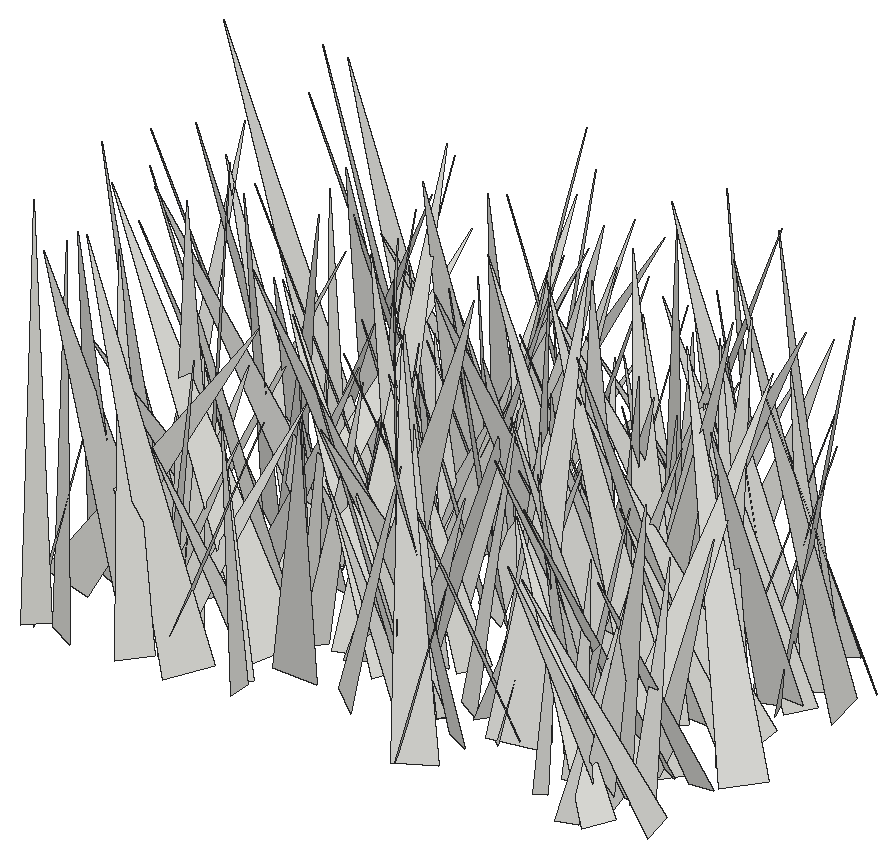
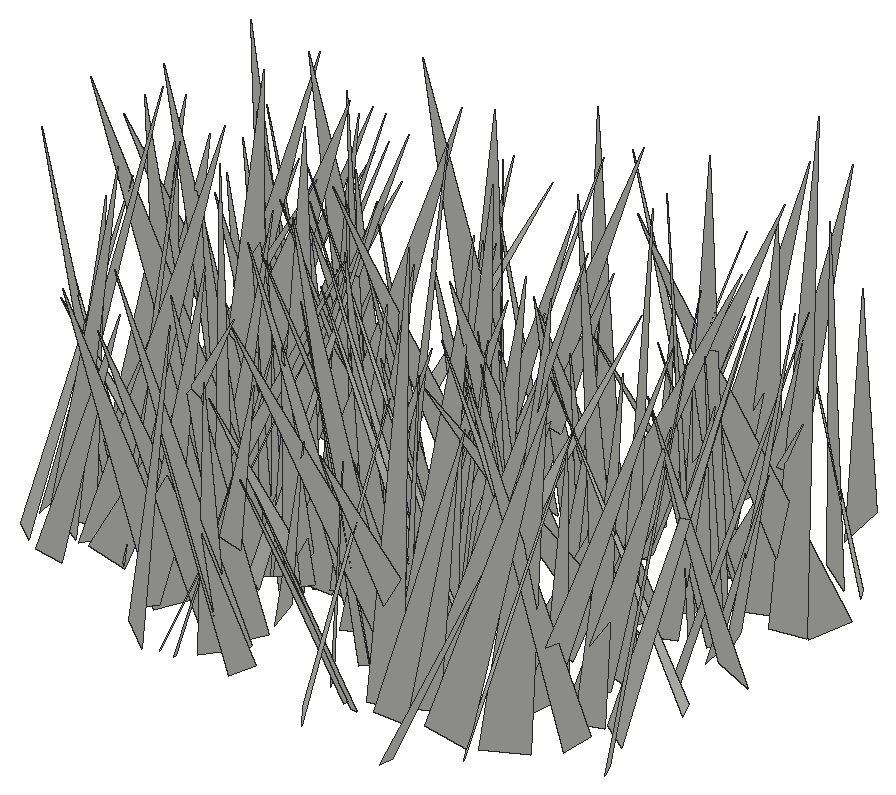
# SketchUp Ruby script. Lengths in inches.
U = 1.inch
M = Sketchup.active_model
def pt(a) = Geom::Point3d.new(a.map { |v| v * U })
def face(e, loops, mat)
  f = e.add_face(loops[0].map { |a| pt(a) })
  loops[1..].each { |l| e.add_face(l.map { |a| pt(a) }).erase! }
  f.material = f.back_material = mat if mat
  f
end
# faces: each face lists its corners as indices into pts; further lists are holes
def faces(e, pts, list, mat = nil) = list.each { |f| face(e, (f[0].is_a?(Array) ? f : [f]).map { |l| l.map { |i| pts[i] } }, mat) }
# xy, xz, yz: faces in a plane at the given z, y or x. An outline is a flat list of corners, or four numbers for a rectangle; further outlines are holes
def ring(l) = l.size == 4 ? [[l[0], l[1]], [l[2], l[1]], [l[2], l[3]], [l[0], l[3]]] : l.each_slice(2).to_a
def flat(e, list, mat, &to3) = list.each { |f| face(e, (f[0].is_a?(Array) ? f : [f]).map { |l| ring(l).map { |u, v| to3.(u, v) } }, mat) }
def xy(e, z, list, mat = nil) = flat(e, list, mat) { |x, y| [x, y, z] }
def xz(e, y, list, mat = nil) = flat(e, list, mat) { |x, z| [x, y, z] }
def yz(e, x, list, mat = nil) = flat(e, list, mat) { |y, z| [x, y, z] }
def lines(e, pts, list) = list.each { |a, b| e.add_line(pt(pts[a]), pt(pts[b])) }
# prism: a flat outline (further loops are holes) pulled along v
def prism(e, loops, v, mat = nil)
  f = face(e, loops, mat); d = Geom::Vector3d.new(v.map { |x| x * U })
  f.pushpull(f.normal.samedirection?(d) ? d.length : -d.length)
end
def box(e, o, s, mat = nil) = prism(e, [[o, [o[0] + s[0], o[1], o[2]], [o[0] + s[0], o[1] + s[1], o[2]], [o[0], o[1] + s[1], o[2]]]], [0, 0, s[2]], mat)
def at(x, y, z, deg = 0) = Geom::Transformation.translation(pt([x, y, z])) * Geom::Transformation.rotation(ORIGIN, Z_AXIS, deg.degrees)
def axes(o, x, y, z) = Geom::Transformation.new([*x, 0, *y, 0, *z, 0, *pt(o).to_a, 1])
def part(name) = M.definitions.add(name)
# library, detail: a bought-in or finely detailed component or shape, given as its bounding box
def library(name, o, s) = part(name).tap { |d| box(d.entities, o, s) }
def detail(e, o, s) = box(e.add_group.entities, o, s)
def put(e, d, t, mat = nil) = e.add_instance(d, t).tap { |i| i.material = mat if mat }
def group(e, t, mat = nil) = e.add_group.tap { |g| g.transformation = t; g.material = mat if mat }.entities
root = M.entities
c1 = part("fur_instance\#9")
p = [[0.8125,0,1.79],[0.67,-0.02,1.48],[0,-0.11,0],[0,0.11,0]]
faces(c1.entities,p,[[0,1,2,3]])
put(root,c1,axes([89.75,154.68,-28.22],[3.15545,2.01724,0.79775],[2.15051,-3.09372,-0.68323],[-0.2846,-1.01105,3.6823]))
put(root,c1,axes([95.03,153.1,-27.1],[-6.05277,2.56522,0.71834],[2.46544,6.06973,-0.90131],[1.00895,0.55714,6.51184]))
put(root,c1,axes([95.66,155,-28.22],[-6.02527,4.37662,1.94606],[4.73834,5.90349,1.39383],[0.70004,-2.28907,7.31546]))
put(root,c1,axes([98.42,156.88,-28.22],[1.84605,-6.6162,0.27609],[-6.51912,-1.76548,1.28157],[1.16252,0.60597,6.74831]))
put(root,c1,axes([93.76,156.59,-28.22],[6.81977,1.54998,0.06465],[1.44583,-6.24479,-2.79788],[0.56233,-2.74155,6.40965]))
put(root,c1,axes([104.08,154.99,-28.22],[3.27913,1.40298,0.59687],[1.4938,-3.23974,-0.59158],[-0.30522,-0.78299,3.51725]))
put(root,c1,axes([91.07,154.34,-28.22],[3.04497,5.63186,2.55497],[5.93211,-3.46487,0.56775],[-1.7481,-1.94792,6.3771]))
put(root,c1,axes([91.22,152.89,-27.1],[-6.67208,0.88571,0.68005],[0.61302,6.34873,-2.25421],[0.93335,2.16166,6.3419]))
put(root,c1,axes([113.36,156.39,-28.22],[-4.90231,-0.23018,0.15933],[-0.18525,4.76264,1.18065],[0.20988,-1.17272,4.76358]))
put(root,c1,axes([111.52,156.59,-28.22],[-4.7933,-0.97536,0.74224],[-0.77682,4.73507,1.20565],[0.94805,-1.05153,4.74061]))
put(root,c1,axes([97.63,155.1,-28.22],[-4.49863,-0.46507,1.40367],[-0.60193,4.68178,-0.37796],[1.35065,0.53749,4.50678]))
put(root,c1,axes([91.66,157.73,-28.22],[5.20163,-5.29224,1.8402],[-4.95757,-5.51713,-1.85336],[-2.61089,-0.0677,7.18539]))
put(root,c1,axes([96.51,157.05,-28.22],[-4.25051,-1.02119,0.70994],[-0.79222,4.17184,1.25768],[0.95876,-1.08007,4.18663]))
put(root,c1,axes([89.99,158.09,-28.22],[-1.25565,-8.18969,1.33935],[-8.04493,1.53362,1.83538],[2.03567,1.00923,8.07955]))
put(root,c1,axes([104.86,154.85,-28.22],[-2.95923,6.17255,1.7602],[6.41346,2.92118,0.53848],[0.25723,-1.82266,6.82403]))
put(root,c1,axes([104.99,156.82,-28.22],[-2.87551,-4.98025,1.4124],[-5.17006,2.84441,-0.49611],[0.26119,1.47404,5.72934]))
put(root,c1,axes([100.61,156.65,-28.22],[3.06956,3.90435,1.71137],[4.25532,-2.68017,-1.51785],[0.25498,-2.27325,4.72887]))
put(root,c1,axes([111.77,155.4375,-28.22],[-3.00277,4.1066,0.06153],[3.92812,2.84936,1.52829],[-1.19912,-0.94951,4.85234]))
put(root,c1,axes([110.73,157.375,-28.22],[1.26894,-6.32164,1.3833],[-6.3592,-0.957,1.46001],[1.19887,1.6149,6.28026]))
put(root,c1,axes([111.05,156.16,-28.22],[4.20018,-2.603,1.54886],[-2.85846,-4.28223,0.55487],[-1.0019,1.30501,4.91012]))
put(root,c1,axes([94.16,155.69,-28.22],[4.52412,1.43506,1.852],[1.32361,-4.8885,0.5546],[-1.93323,0.01133,4.71375]))
put(root,c1,axes([93.89,156.42,-28.22],[-2.52559,2.65872,0.46687],[2.62617,2.27215,1.26725],[-0.62447,-1.19747,3.44114]))
put(root,c1,axes([97.36,155.55,-28.22],[-3.44021,1.49763,0.22694],[1.46636,3.43395,-0.43273],[0.37973,0.30751,3.72702]))
put(root,c1,axes([109.33,157.41,-28.22],[-1.75963,-5.21212,1.71135],[-5.46295,1.82898,-0.04671],[0.50104,1.63703,5.50093]))
put(root,c1,axes([103.04,157.14,-28.22],[-5.74367,-4.09689,1.01684],[-4.21686,5.6466,-1.0688],[0.19121,1.46278,6.97366]))
put(root,c1,axes([110.91,154.9,-28.22],[-3.77654,1.99621,0.89861],[1.50689,3.67022,-1.82025],[1.58796,1.26459,3.86442]))
put(root,c1,axes([89.07,157.1,-28.22],[3.63581,-6.29578,1.08718],[-5.74464,-2.67402,3.72648],[2.79605,2.69271,6.24254]))
put(root,c1,axes([92.64,157.16,-28.22],[2.90459,3.11145,0.76807],[3.13189,-2.53582,-1.57117],[0.67994,-1.61126,3.9559]))
put(root,c1,axes([109.1,157.25,-28.22],[4.01593,3.70117,1.52807],[3.99587,-3.8439,-1.19115],[-0.25835,-1.92018,5.32987]))
put(root,c1,axes([111.21,159.3,-28.22],[-1.38983,-5.84462,0.0201],[-5.82782,1.38425,-0.46046],[-0.44334,0.12603,5.98992]))
put(root,c1,axes([109.51,157.06,-28.22],[0.95056,-3.70171,1.6828],[-4.06505,-0.90725,0.30052],[-0.09921,1.70654,3.80998]))
put(root,c1,axes([94.23,155.71,-28.22],[1.65691,4.63189,0.02775],[4.518,-1.60961,-1.09423],[1.0212,-0.39403,4.79608]))
put(root,c1,axes([102.22,157.55,-28.22],[-3.97846,-0.22397,0.26493],[-0.21326,3.98441,0.16592],[0.27363,-0.15114,3.9813]))
put(root,c1,axes([103.54,157.51,-28.22],[-1.39517,3.65073,1.37856],[3.73252,0.82124,1.60268],[-1.13865,-1.78115,3.56451]))
put(root,c1,axes([97.07,157.6,-28.22],[-7.15301,3.97515,0.71331],[4.02795,6.91641,1.848],[-0.2937,-1.95899,7.97197]))
put(root,c1,axes([112.79,159.31,-28.22],[-0.25255,-4.7231,0.0991],[-4.68784,0.23828,-0.59045],[-0.58449,0.12972,4.69284]))
put(root,c1,axes([112.24,157.03,-28.22],[0.04059,4.23783,1.33242],[4.44047,0.00019,-0.13586],[0.12965,-1.33303,4.23585]))
put(root,c1,axes([109.14,155.79,-28.22],[1.37607,4.21587,0.41156],[3.82506,-1.42264,1.78368],[-1.81985,0.19763,4.06025]))
put(root,c1,axes([106.23,158.34,-28.22],[-5.23491,-4.53939,0.15815],[-4.43832,5.06084,-1.65066],[-0.96564,1.34804,6.72946]))
put(root,c1,axes([103.45,157.3125,-28.22],[-4.02288,2.74208,1.38872],[2.85785,4.17888,0.02734],[1.13147,-0.80565,4.86845]))
put(root,c1,axes([108.68,159.2,-28.22],[3.89618,-1.88557,1.1779],[-1.51971,-3.99347,-1.36592],[-1.62275,-0.78732,4.1073]))
put(root,c1,axes([93,158.62,-28.22],[6.49174,-3.69034,2.54193],[-3.75607,-6.92147,-0.45599],[-2.44375,0.83512,7.45341]))
put(root,c1,axes([110.06,158.83,-28.22],[-6.30832,-1.1114,1.05664],[-1.00602,6.37534,0.69964],[1.15742,-0.51611,6.36715]))
put(root,c1,axes([94.56,156.49,-28.22],[-4.63028,1.37895,0.71291],[1.15549,4.55932,-1.31404],[1.03661,1.07721,4.64912]))
put(root,c1,axes([110.44,159.28,-28.22],[-1.67937,-5.43767,0.87836],[-5.25266,1.30456,-1.96667],[-1.65811,1.37475,5.34049]))
put(root,c1,axes([101.4,158.98,-28.22],[3.13596,-3.23192,0.2957],[-3.22644,-3.06024,0.76944],[0.35051,0.74607,4.43707]))
put(root,c1,axes([99.68,159.16,-28.22],[6.25642,-5.32962,1.03257],[-5.42827,-6.12142,1.29455],[0.06986,1.65444,8.11614]))
put(root,c1,axes([100.4,161.69,-28.22],[5.3138,-2.81187,1.14067],[-1.98861,-4.96443,-2.9739],[-2.29198,-2.2118,5.22484]))
put(root,c1,axes([105.83,157.65,-28.22],[2.60004,3.22909,0.64132],[3.22546,-2.66223,0.32783],[-0.65933,-0.2899,4.13277]))
put(root,c1,axes([100.03,161.35,-28.22],[-0.28332,-7.79704,0.77926],[-7.68212,0.12267,-1.56569],[-1.54472,0.82004,7.64347]))
put(root,c1,axes([111.26,158.86,-28.22],[4.23339,-1.74729,1.15695],[-1.93705,-4.25778,0.65751],[-0.79963,1.0637,4.53236]))
put(root,c1,axes([100.9,158.96,-28.22],[4.97701,4.02381,2.97396],[4.34378,-5.5566,0.24873],[-2.48337,-1.65505,6.3953]))
put(root,c1,axes([96.49,159.06,-28.22],[-7.32124,-3.15954,0.71739],[-3.23761,7.2018,-1.32279],[0.12329,1.49974,7.86343]))
put(root,c1,axes([97.66,158.77,-28.22],[4.38322,-1.64948,1.59394],[-1.93146,-4.50849,0.64578],[-1.2373,1.19448,4.63858]))
put(root,c1,axes([106.49,157.76,-28.22],[-2.78975,7.45432,2.27613],[7.61508,3.12201,-0.8911],[1.66081,-1.79348,7.90921]))
put(root,c1,axes([107,158.4,-28.22],[-1.61358,3.38665,0.61033],[3.4322,1.63258,0.01498],[0.24881,-0.55751,3.75138]))
put(root,c1,axes([90.68,162.89,-28.22],[-5.2943,-3.28141,1.0592],[-2.29433,4.80125,3.40634],[2.57403,-2.46971,5.21479]))
put(root,c1,axes([104,158.61,-28.22],[2.52877,4.50107,1.40807],[4.66336,-2.62485,0.01569],[-0.70386,-1.21962,5.16276]))
put(root,c1,axes([104.61,160.28,-28.22],[3.51068,-4.45404,1.06123],[-4.56743,-3.50052,0.41776],[-0.32136,1.09429,5.65587]))
put(root,c1,axes([101.22,160.06,-28.22],[1.40139,-5.88916,2.09043],[-6.21682,-1.53152,-0.14692],[-0.635,1.99706,6.05182]))
put(root,c1,axes([104.79,158.55,-28.22],[5.00649,-0.69371,1.01239],[-0.92226,-4.93206,1.18126],[-0.80969,1.32843,4.91435]))
put(root,c1,axes([100.7,159.03,-28.22],[-4.99082,4.3261,0.4502],[4.29852,4.80129,1.51542],[-0.66378,-1.43477,6.4286]))
put(root,c1,axes([96.7,159.86,-28.22],[-3.86454,-2.68359,1.87384],[-2.96857,4.09497,-0.25773],[1.3786,1.29506,4.69786]))
put(root,c1,axes([111.6,159.08,-28.22],[-2.9065,7.574,1.65107],[7.44857,2.24028,2.83534],[-2.14716,-2.4809,7.60092]))
put(root,c1,axes([92.16,160.19,-28.22],[6.26613,3.81902,2.82967],[4.24719,-6.60086,-0.4964],[-2.13385,-1.92357,7.3214]))
put(root,c1,axes([91.94,159.12,-28.22],[-4.86729,-1.78674,2.25978],[-2.35287,5.02555,-1.09424],[1.66225,1.88173,5.06809]))
put(root,c1,axes([96.64,159.73,-28.22],[4.11345,0.18865,1.81103],[0.00918,-4.47631,0.44541],[-1.8208,0.4036,4.09361]))
put(root,c1,axes([91.16,160.11,-28.22],[0.33455,3.97904,1.71347],[4.11253,0.24873,-1.38056],[1.36232,-1.72801,3.74683]))
put(root,c1,axes([93.95,160.3,-28.22],[4.93305,-2.19664,0.15391],[-2.18894,-4.85066,0.92924],[0.23965,0.9109,5.31946]))
put(root,c1,axes([90.83,159.85,-28.22],[-6.73527,-1.87686,1.53677],[-2.12146,6.75676,-1.04577],[1.17629,1.43931,6.91323]))
put(root,c1,axes([110.32,162.51,-28.22],[-0.93689,-7.58778,0.99671],[-7.63501,0.85799,-0.64504],[-0.52389,1.06539,7.61814]))
put(root,c1,axes([102.55,160.74,-28.22],[-3.29735,3.76242,1.32483],[3.9802,2.99017,1.41439],[-0.2628,-1.92005,4.79874]))
put(root,c1,axes([112.62,161.26,-28.22],[-4.62797,0.36048,0.06702],[0.36662,4.56134,0.78248],[0.00509,-0.78533,4.57556]))
put(root,c1,axes([110.4375,158.32,-28.22],[-1.75958,6.89289,0.89816],[6.66639,1.93582,-1.79628],[1.96924,-0.39424,6.88342]))
put(root,c1,axes([90.89,160.72,-28.22],[-3.86057,-0.50737,0.50019],[-0.53854,3.88252,-0.21837],[0.46646,0.28336,3.88764]))
put(root,c1,axes([102.22,158.06,-28.22],[7.12647,2.20024,1.82821],[1.44023,-6.99989,2.8102],[-2.47167,2.26505,6.90872]))
put(root,c1,axes([108.63,160.82,-28.22],[-8.06825,0.70999,0.37952],[0.71569,8.07597,0.10667],[0.36866,-0.13964,8.09873]))
put(root,c1,axes([95.95,162.07,-28.22],[-0.05824,-3.81958,0.55077],[-3.85535,0.08183,0.15984],[0.16986,0.54776,3.81668]))
put(root,c1,axes([104.04,161.77,-28.22],[7.07527,1.73735,2.55738],[2.12787,-7.36989,-0.88027],[-2.24293,-1.5114,7.23207]))
put(root,c1,axes([92.92,160.8,-28.22],[-3.33055,3.67395,0.98734],[3.8043,3.21801,0.85849],[0.0046,-1.30837,4.884]))
put(root,c1,axes([104.76,161.06,-28.22],[1.88047,-2.78184,1.95652],[-3.20631,-2.19563,-0.04014],[-1.13412,1.59479,3.35756]))
put(root,c1,axes([113.75,160.25,-28.22],[-4.84886,5.21937,0.60309],[5.25064,4.78392,0.8135],[-0.19034,-0.99462,7.07753]))
put(root,c1,axes([112.51,162.64,-28.22],[-6.49837,1.01991,0.13564],[1.01971,6.26851,1.71854],[-0.13717,-1.71841,6.34946]))
put(root,c1,axes([106.7,161.48,-28.22],[4.67154,-2.82363,0.84685],[-2.94301,-4.55853,1.0353],[-0.16964,1.32674,5.35951]))
put(root,c1,axes([95.23,163.375,-28.22],[0.24896,-7.3468,1.55373],[-6.97419,-0.80255,-2.67734],[-2.78393,1.35351,6.84612]))
put(root,c1,axes([106.46,163.44,-28.22],[-0.95692,-4.60949,0.0097],[-4.59629,0.95343,-0.35816],[-0.34872,0.08227,4.69412]))
put(root,c1,axes([91.27,164.24,-28.22],[-5.06426,-4.56399,0.84014],[-4.29824,5.08189,1.69768],[1.74956,-0.72593,6.60262]))
put(root,c1,axes([103.72,165.08,-28.22],[1.8393,-7.94223,0.20343],[-7.82957,-1.84746,-1.33722],[-1.34842,-0.10629,8.04201]))
put(root,c1,axes([91.95,163.83,-28.22],[-3.33298,-6.74445,1.96036],[-6.484,3.7887,2.01069],[2.69971,0.77298,7.24938]))
put(root,c1,axes([100.91,164.12,-28.22],[-3.9717,-6.10655,1.7462],[-5.81347,4.32471,1.90107],[2.55787,0.34722,7.03209]))
put(root,c1,axes([109.38,161.49,-28.22],[-5.36752,5.77658,2.45123],[6.12108,5.53013,0.37117],[1.38195,-2.05828,7.87664]))
put(root,c1,axes([100.49,161.9375,-28.22],[-0.11529,-4.79427,2.44231],[-5.06003,0.9271,1.58106],[1.8292,2.26244,4.52754]))
put(root,c1,axes([92.68,163.7,-28.22],[7.66875,0.29762,1.40281],[0.64374,-7.5341,-1.92071],[-1.28143,-2.00373,7.43029]))
put(root,c1,axes([104.48,159.58,-28.22],[3.19327,6.60837,0.52108],[6.51338,-3.23542,1.11669],[-1.23207,0.02336,7.254]))
put(root,c1,axes([97.54,162.26,-28.22],[3.79573,2.84609,1.46317],[3.05532,-3.89817,-0.34352],[-0.95191,-1.16307,4.73179]))
put(root,c1,axes([112.92,160.89,-28.22],[-0.8728,6.82324,1.17968],[6.78553,0.6058,1.51645],[-1.38016,-1.33658,6.7096]))
put(root,c1,axes([111.5,164.94,-28.22],[2.0561,-6.44135,0.2848],[-6.4395,-2.06652,-0.24899],[-0.32395,0.19535,6.75697]))
put(root,c1,axes([107.68,162.73,-28.22],[7.40162,-2.04644,1.37858],[-2.14984,-7.48787,0.42713],[-1.21103,0.78507,7.66743]))
put(root,c1,axes([102.92,164.84,-28.22],[0.94954,-6.1364,0.24208],[-6.03443,-0.88683,1.18943],[1.14,0.41683,6.09444]))
put(root,c1,axes([98.21,163.19,-28.22],[-4.53938,3.59005,2.40826],[4.08452,4.7056,0.68422],[1.41595,-2.06469,5.74685]))
put(root,c1,axes([98.53,162.81,-28.22],[-5.69424,-4.56861,0.52497],[-4.47673,5.31586,-2.29625],[-1.05201,2.10752,6.92992]))
put(root,c1,axes([104.88,165.31,-28.22],[-1.64763,-7.14584,1.34901],[-6.49832,2.06763,3.01567],[3.26416,0.50931,6.68457]))
put(root,c1,axes([100.79,163.62,-28.22],[-3.66395,-2.75565,0.79106],[-2.79858,3.7164,-0.01609],[0.62239,0.48852,4.58453]))
put(root,c1,axes([99.1,159.17,-28.22],[-7.03666,4.34174,0.35439],[3.96979,6.66848,-2.87454],[1.79361,2.2741,7.75256]))
put(root,c1,axes([103.86,165.39,-28.22],[0.44147,-7.17503,0.62576],[-6.54369,-0.13768,3.03788],[3.00878,0.75334,6.51516]))
put(root,c1,axes([105.21,165.03,-28.22],[2.17041,-4.52553,0.56409],[-4.42394,-2.24099,-0.95709],[-1.10786,0.0828,4.92697]))
put(root,c1,axes([108.24,163.66,-28.22],[-5.73495,-0.11109,1.68244],[-0.04447,5.97258,0.24275],[1.68552,-0.22038,5.73089]))
put(root,c1,axes([110.04,163.16,-28.22],[4.86014,-4.74094,2.82615],[-5.30574,-5.05065,0.65171],[-1.52079,2.46963,6.75816]))
put(root,c1,axes([103.17,163.16,-28.22],[-3.65531,3.57205,1.42816],[3.77376,3.712,0.37448],[0.74692,-1.27356,5.09712]))
put(root,c1,axes([104.31,164.8125,-28.22],[4.53182,-5.76132,1.66498],[-5.89155,-4.66684,-0.11276],[-1.12014,1.237,7.32923]))
put(root,c1,axes([105.14,165.9375,-28.22],[-4.06699,-5.2197,0.56162],[-5.13541,4.10303,0.94539],[1.09007,-0.14467,6.54919]))
put(root,c1,axes([97.29,162.29,-28.22],[-5.55203,-0.57439,2.02149],[-1.15794,5.60149,-1.58866],[1.75372,1.88009,5.3508]))
put(root,c1,axes([99.27,163.22,-28.22],[-5.21816,-1.76906,1.50642],[-2.07355,5.2165,-1.05669],[1.04846,1.51216,5.4076]))
put(root,c1,axes([106.38,165.03,-28.22],[1.53942,-5.44162,0.89342],[-5.38829,-1.28703,1.44538],[1.17292,1.22946,5.46735]))
put(root,c1,axes([89.66,161.25,-28.22],[1.53889,6.65129,0.3221],[6.53467,-1.57198,1.24039],[-1.28121,-0.02868,6.71336]))
put(root,c1,axes([100.54,166.38,-28.22],[4.29462,-4.11505,0.26594],[-3.98176,-4.23808,-1.27765],[-1.07236,-0.74374,5.80905]))
put(root,c1,axes([89.41,163.93,-28.22],[5.0651,3.0377,0.15182],[3.00547,-4.95362,-1.15532],[0.46672,-1.0677,5.79207]))
put(root,c1,axes([102.14,165.07,-28.22],[-1.57238,-4.56901,1.11948],[-4.65933,1.35009,-1.0341],[-0.64787,1.37945,4.72005]))
put(root,c1,axes([91.16,166.56,-28.22],[-0.0268,-5.65268,0.22398],[-5.53849,0.07185,1.15049],[1.15241,0.21383,5.53443]))
put(root,c1,axes([105.64,165.125,-28.22],[6.6749,-4.96789,0.00129],[-4.8195,-6.47499,2.02019],[1.20515,1.62135,8.07174]))
put(root,c1,axes([90.12,166.6,-28.22],[-4.17901,-5.88434,0.7845],[-5.89024,4.22956,0.34775],[0.73891,0.43633,7.20893]))
put(root,c1,axes([93.92,161.59,-28.22],[-1.93127,6.17376,0.09606],[5.65668,1.80943,-2.5656],[2.47519,0.68189,5.93825]))
put(root,c1,axes([98.02,164.98,-28.22],[3.07396,-3.53335,0.83024],[-3.61315,-2.87553,1.13994],[0.34489,1.36741,4.5425]))
put(root,c1,axes([112.19,165.05,-28.22],[-2.9134,4.03937,1.46912],[4.26943,2.51447,1.5531],[-0.49677,-2.07934,4.73205]))
put(root,c1,axes([96.58,165.56,-28.22],[7.11507,4.33314,0.48127],[4.20256,-6.57141,-2.9643],[1.16029,-2.76992,7.78545]))
put(root,c1,axes([113.28,165.86,-28.22],[-7.78363,-1.77881,1.5879],[-1.77027,7.9428,0.22014],[1.59741,0.13482,7.98126]))
put(root,c1,axes([92.41,164.95,-28.22],[-5.38349,2.8617,0.60302],[2.91403,5.35589,0.59819],[0.24775,-0.81245,6.06741]))
put(root,c1,axes([109.96,165.5,-28.22],[4.56554,2.4835,0.72557],[2.58092,-4.47494,-0.92307],[-0.18188,-1.15993,5.11467]))
put(root,c1,axes([88.92,168.48,-28.22],[-6.01376,-4.74049,2.00405],[-3.98095,6.23797,2.80955],[3.26197,-1.12665,7.12348]))
put(root,c1,axes([97.99,165.38,-28.22],[1.74245,-3.02379,2.07472],[-3.3962,-2.19711,-0.34987],[-1.38332,1.58534,3.47232]))
put(root,c1,axes([99.85,165.86,-28.22],[-0.07815,-6.05054,2.52953],[-6.4447,0.53908,1.09033],[1.2138,2.47266,5.952]))
put(root,c1,axes([104.13,164.875,-28.22],[-3.32764,3.062,1.30373],[3.08153,3.53122,-0.42827],[1.25687,-0.55083,4.50173]))
put(root,c1,axes([94.69,164.78,-28.22],[4.79862,3.05458,1.6678],[3.017,-5.06719,0.60002],[-1.73486,-0.36311,5.65661]))
put(root,c1,axes([111.5,164.89,-28.22],[6.18065,2.99725,1.89028],[2.99834,-6.44896,0.42186],[-1.88855,-0.42956,6.85609]))
put(root,c1,axes([106.61,166.26,-28.22],[-2.89308,-3.13599,0.85003],[-3.23039,2.89836,-0.3018],[0.34876,0.83187,4.25597]))
put(root,c1,axes([110.29,163.35,-28.22],[4.22042,3.02936,0.44277],[2.70703,-4.0447,1.87014],[-1.43005,1.2839,4.84681]))
put(root,c1,axes([107.19,167.35,-28.22],[-6.50951,0.22142,0.60358],[0.38251,6.26967,1.82536],[0.51674,-1.85181,6.25226]))
put(root,c1,axes([95.17,163.46,-28.22],[5.52585,4.05046,1.31825],[3.69086,-5.63091,1.83015],[-2.12639,0.75214,6.60241]))
put(root,c1,axes([98.92,166.5,-28.22],[2.58883,2.26123,2.35644],[2.87323,-3.00647,-0.27159],[-1.55259,-1.79333,3.42658]))
put(root,c1,axes([100.75,163.76,-28.22],[3.08355,6.47581,0.56476],[6.50039,-3.07095,-0.27862],[0.00972,-0.62967,7.16706]))
put(root,c1,axes([99.5,164.01,-28.22],[6.38887,5.18246,1.59043],[5.07791,-6.58181,1.04866],[-1.89794,-0.16426,8.1594]))
put(root,c1,axes([112.77,167.89,-28.22],[-3.86726,-4.8383,0.71579],[-4.78645,3.93151,0.71436],[1.00566,0.10641,6.1526]))
put(root,c1,axes([111.9,166.4,-28.22],[1.93856,-5.12728,2.24723],[-5.46022,-2.25638,-0.43794],[-1.23493,1.9279,5.46399]))
put(root,c1,axes([109.43,167.22,-28.22],[4.54557,4.08977,3.87164],[5.12111,-5.0718,-0.65499],[-2.34307,-3.15097,6.07942]))
put(root,c1,axes([101.04,165.73,-28.22],[6.39922,1.66084,0.77373],[1.68967,-6.43637,-0.15871],[-0.70856,-0.34898,6.60932]))
put(root,c1,axes([96.375,167.8,-28.22],[-4.58981,-6.81856,1.14154],[-6.9132,4.53833,-0.68805],[0.05895,1.33156,8.19058]))
put(root,c1,axes([93.76,164.9375,-28.22],[1.02305,5.31057,1.33507],[5.15193,-1.39366,1.59576],[-1.8553,-0.94167,5.16743]))
put(root,c1,axes([110.54,166.73,-28.22],[-7.81883,2.51294,1.68172],[2.76611,7.82758,1.16397],[1.22135,-1.64052,8.12983]))
put(root,c1,axes([98.28,167.49,-28.22],[-2.51428,-3.3921,0.48717],[-3.39486,2.54791,0.21985],[0.4675,0.25907,4.21659]))
put(root,c1,axes([96.53,166.76,-28.22],[6.0574,2.72005,0.2303],[2.69232,-5.86042,-1.5971],[0.45071,-1.54939,6.44516]))
put(root,c1,axes([96.19,169.16,-28.22],[5.05065,-5.78899,0.88016],[-5.66798,-5.12516,-1.18448],[-1.47008,-0.1285,7.59069]))
put(root,c1,axes([98.44,166.83,-28.22],[4.08139,-3.20586,0.61223],[-3.2526,-3.91407,1.18774],[0.27008,1.30866,5.05219]))
put(root,c1,axes([98.7,167.64,-28.22],[1.53835,-7.01276,2.03333],[-7.04829,-0.88366,2.28484],[1.90652,2.39168,6.80623]))
put(root,c1,axes([97.71,167.65,-28.22],[-2.86919,-3.90872,1.79506],[-4.01549,3.2075,0.56601],[1.54149,1.08002,4.8156]))
put(root,c1,axes([92.19,169.54,-28.22],[4.1786,-6.03386,0.40804],[-6.0035,-4.19846,-0.60465],[-0.72937,-0.01047,7.31455]))
put(root,c1,axes([93.0625,166.99,-28.22],[-8.2127,0.65784,0.53458],[0.66874,8.22786,0.14871],[0.52088,-0.19122,8.23766]))
put(root,c1,axes([104.6,168.03,-28.22],[7.08469,1.17747,2.52447],[1.61288,-7.35894,-1.094],[-2.27113,-1.55299,7.09806]))
put(root,c1,axes([93.11,169.34,-28.22],[-2.96228,-3.48582,0.87467],[-2.85625,2.97145,2.16874],[2.18125,-0.843,4.02773]))
put(root,c1,axes([104.45,167.8,-28.22],[3.92592,-0.41216,0.89749],[-0.2951,-4.00034,-0.54626],[-0.94248,-0.46433,3.90952]))
put(root,c1,axes([112.15,166.75,-28.22],[1.97558,6.78512,3.04566],[6.89111,-2.85534,1.89119],[-2.79761,-2.24188,6.80913]))
put(root,c1,axes([104.09,164.67,-28.22],[4.15865,3.49208,0.81847],[2.77358,-3.92559,2.6563],[-2.27416,1.59814,4.73636]))
put(root,c1,axes([96.95,169.59,-28.22],[-0.53699,-7.34105,1.16615],[-7.27133,0.76139,1.44476],[1.5423,1.0337,7.21748]))
put(root,c1,axes([90.71,167.73,-28.22],[6.32916,0.13104,0.27334],[0.13733,-6.3333,-0.14369],[-0.27023,-0.14945,6.32889]))
put(root,c1,axes([109.73,167.57,-28.22],[-2.44299,5.49091,1.30941],[5.27932,1.71736,2.64808],[-1.99837,-2.17564,5.395]))
put(root,c1,axes([111.1875,168.66,-28.22],[0.38107,-4.3176,1.24457],[-4.35966,-0.65774,-0.94692],[-1.08815,1.12319,4.22969]))
put(root,c1,axes([103.08,167.03,-28.22],[-4.4304,-0.23548,0.66281],[-0.42328,4.26855,-1.31284],[0.56178,1.35914,4.23796]))
put(root,c1,axes([102.96,168.88,-28.22],[4.31446,-3.71791,0.40504],[-3.72385,-4.21342,0.9907],[0.3462,1.01276,5.60856]))
put(root,c1,axes([99.55,167.2,-28.22],[-4.49953,-3.59508,3.80394],[-4.60675,5.10137,-0.62788],[2.48443,2.94818,5.72505]))
put(root,c1,axes([106.68,169.125,-28.22],[4.62611,-3.05223,2.53258],[-2.97331,-5.24406,-0.88892],[-2.62479,0.5609,5.47054]))
put(root,c1,axes([104.66,168.3,-28.22],[1.4221,-3.78822,2.5832],[-4.25079,-2.10312,-0.74405],[-1.71882,2.06693,3.97736]))
put(root,c1,axes([104.8,170.97,-28.22],[-4.66281,-2.88259,0.04543],[-2.761,4.48988,1.50703],[0.82963,-1.25893,5.27068]))
put(root,c1,axes([96.75,167.9,-28.22],[6.3813,-2.25892,0.20905],[-2.20352,-6.02357,2.17449],[0.53935,2.11689,6.41056]))
put(root,c1,axes([104.35,168.73,-28.22],[3.58397,-3.64133,0.7361],[-3.60405,-3.15993,1.91614],[0.90107,1.84433,4.7363]))
put(root,c1,axes([96.37,170.09,-28.22],[0.91416,-4.94391,1.27953],[-4.9749,-1.15567,-0.91103],[-1.1532,1.06645,4.94449]))
put(root,c1,axes([104.1,171.2,-28.22],[-3.17214,-2.54983,0.51656],[-2.07776,2.97317,1.9168],[1.56569,-1.22048,3.59026]))
put(root,c1,axes([99.27,169.33,-28.22],[2.96101,1.91002,1.7712],[2.18546,-3.28075,-0.11568],[-1.41742,-1.06838,3.5217]))
put(root,c1,axes([106.22,168.67,-28.22],[3.63193,-4.05591,1.60644],[-4.34601,-3.18259,1.79036],[0.37856,2.37544,5.14159]))
put(root,c1,axes([97.58,166.54,-28.22],[-4.47907,3.89554,0.463],[3.44419,4.24137,-2.36643],[1.87807,1.51235,5.44401]))
put(root,c1,axes([98.03,170.13,-28.22],[2.45066,3.05169,0.44917],[2.65928,-1.79957,-2.28257],[1.56295,-1.7231,3.17938]))
put(root,c1,axes([103.3,170.28,-28.22],[3.58428,-2.61771,1.24135],[-2.70899,-3.7283,-0.04015],[-1.02701,0.69843,4.43823]))
put(root,c1,axes([94.2,169.96,-28.22],[0.18988,-6.4583,3.19895],[-6.79344,-1.22898,-2.07794],[-2.40669,2.95955,6.11783]))
put(root,c1,axes([93.42,169.87,-28.22],[-6.3033,-3.29184,1.05702],[-3.45211,6.11366,-1.54635],[0.19083,1.86335,6.94094]))
put(root,c1,axes([101.86,170.61,-28.22],[3.34433,-2.45993,0.06359],[-2.39384,-3.22746,1.0454],[0.56992,0.87868,4.01783]))
put(root,c1,axes([102.49,169.92,-28.22],[6.76067,1.19839,0.69108],[1.18973,-6.79585,0.14582],[-0.7059,0.02372,6.86451]))
put(root,c1,axes([97.55,170.4,-28.22],[2.51119,2.94201,0.30611],[2.79372,-2.22715,-1.51331],[0.97173,-1.19981,3.55969]))
put(root,c1,axes([94.7,172.33,-28.22],[-4.59731,-1.23154,0.33008],[-1.08177,4.4213,1.42926],[0.67485,-1.30242,4.53973]))
put(root,c1,axes([98.59,171.7,-28.22],[-4.48858,-3.56813,1.07524],[-3.58767,4.5928,0.2643],[1.00813,0.45789,5.72792]))
put(root,c1,axes([105.93,170.875,-28.22],[-3.8782,-4.63911,2.52217],[-5.26639,3.62608,-1.42825],[0.38461,2.87286,5.87554]))
